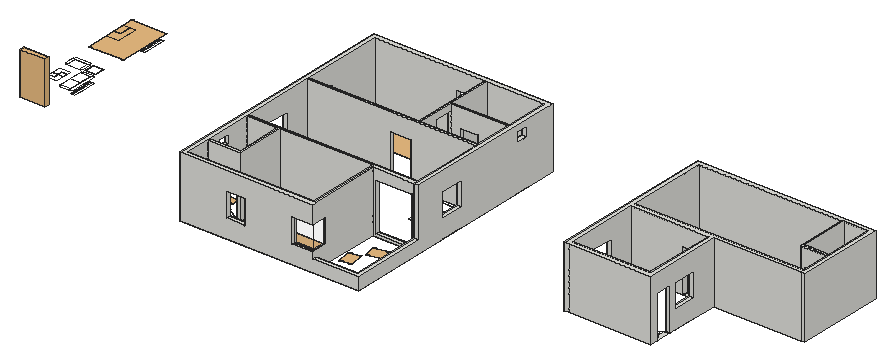
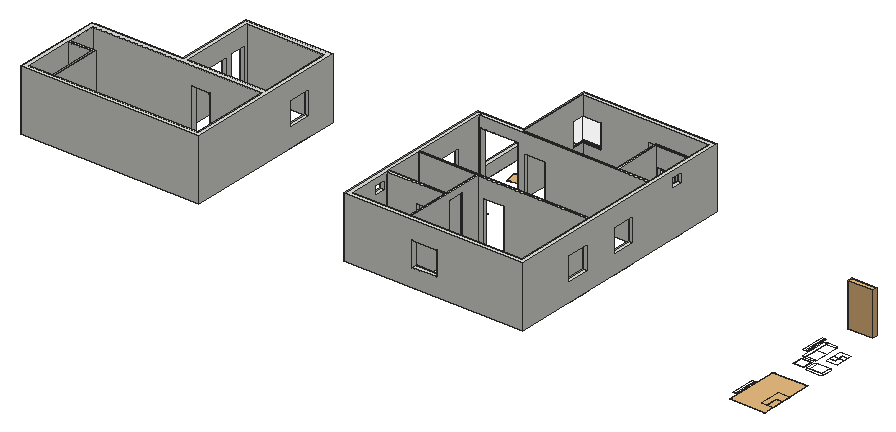
# SketchUp Ruby script. Lengths in inches.
U = 1.inch
M = Sketchup.active_model
def pt(a) = Geom::Point3d.new(a.map { |v| v * U })
def face(e, loops, mat)
  f = e.add_face(loops[0].map { |a| pt(a) })
  loops[1..].each { |l| e.add_face(l.map { |a| pt(a) }).erase! }
  f.material = f.back_material = mat if mat
  f
end
# faces: each face lists its corners as indices into pts; further lists are holes
def faces(e, pts, list, mat = nil) = list.each { |f| face(e, (f[0].is_a?(Array) ? f : [f]).map { |l| l.map { |i| pts[i] } }, mat) }
# xy, xz, yz: faces in a plane at the given z, y or x. An outline is a flat list of corners, or four numbers for a rectangle; further outlines are holes
def ring(l) = l.size == 4 ? [[l[0], l[1]], [l[2], l[1]], [l[2], l[3]], [l[0], l[3]]] : l.each_slice(2).to_a
def flat(e, list, mat, &to3) = list.each { |f| face(e, (f[0].is_a?(Array) ? f : [f]).map { |l| ring(l).map { |u, v| to3.(u, v) } }, mat) }
def xy(e, z, list, mat = nil) = flat(e, list, mat) { |x, y| [x, y, z] }
def xz(e, y, list, mat = nil) = flat(e, list, mat) { |x, z| [x, y, z] }
def yz(e, x, list, mat = nil) = flat(e, list, mat) { |y, z| [x, y, z] }
def lines(e, pts, list) = list.each { |a, b| e.add_line(pt(pts[a]), pt(pts[b])) }
# prism: a flat outline (further loops are holes) pulled along v
def prism(e, loops, v, mat = nil)
  f = face(e, loops, mat); d = Geom::Vector3d.new(v.map { |x| x * U })
  f.pushpull(f.normal.samedirection?(d) ? d.length : -d.length)
end
def box(e, o, s, mat = nil) = prism(e, [[o, [o[0] + s[0], o[1], o[2]], [o[0] + s[0], o[1] + s[1], o[2]], [o[0], o[1] + s[1], o[2]]]], [0, 0, s[2]], mat)
def at(x, y, z, deg = 0) = Geom::Transformation.translation(pt([x, y, z])) * Geom::Transformation.rotation(ORIGIN, Z_AXIS, deg.degrees)
def axes(o, x, y, z) = Geom::Transformation.new([*x, 0, *y, 0, *z, 0, *pt(o).to_a, 1])
def part(name) = M.definitions.add(name)
# library, detail: a bought-in or finely detailed component or shape, given as its bounding box
def library(name, o, s) = part(name).tap { |d| box(d.entities, o, s) }
def detail(e, o, s) = box(e.add_group.entities, o, s)
def put(e, d, t, mat = nil) = e.add_instance(d, t).tap { |i| i.material = mat if mat }
def group(e, t, mat = nil) = e.add_group.tap { |g| g.transformation = t; g.material = mat if mat }.entities
root = M.entities
M.materials.add("[Translucent Glass Gray]").color = [128, 128, 128]
M.materials["[Translucent Glass Gray]"].alpha = 0.1
c1 = part("TABLE 2")
p = [[18.6875,1.33,0],[-2.65,1.33,0],[-2.65,-10.67,0],[-18.65,-10.67,0],[-18.6875,10.67,0],[18.6875,10.67,0],
  [18.6875,0,0],[18.6875,-10.67,0],[-1.28,-10.67,0],[-1.28,0,0]]
lines(c1.entities,p,[[0,1],[1,2],[2,3],[3,4],[4,5],[5,0],[6,7],[7,8],[8,9],[9,6]])
c2 = part("A$C03AA15B9")
p = [[12,-9.82,0],[0,-9.82,0],[0,-0.97,0],[12,-0.97,0],[-1.19,-0.97,0],[-1.19,-10.64,0],
  [12,-10.64,0],[12,-19.5,0],[-12,-19.5,0],[-12,-0.97,0],[-12,9.45,0],[0,9.45,0],
  [0,0.22,0],[-12,0.22,0],[1.19,0.22,0],[1.19,10.64,0],[-12,10.64,0],[-12,19.5,0],
  [12,19.5,0],[12,0.22,0]]
lines(c2.entities,p,[[0,1],[1,2],[2,3],[3,0],[4,5],[5,6],[6,7],[7,8],[8,9],[9,4],[10,11],[11,12],
  [12,13],[13,10],[14,15],[15,16],[16,17],[17,18],[18,19],[19,14]])
c3 = part("A$C47E27A62")
p = [[17.04,-15,0],[-17.04,-15,0],[-17.04,-12,0],[17.04,8.51,0],[-17.04,8.51,0],[17.04,15,0],
  [-17.04,15,0],[13.4375,7.07,0],[-13.4375,7.07,0],[-17.04,9.96,0],[-19.5625,9.96,0],[-19.5625,-12,0],
  [-13.4375,-12,0],[-13.4375,8.51,0],[17.04,-12,0],[17.04,9.96,0],[19.5625,9.96,0],[19.5625,-12,0],
  [13.4375,-12,0],[13.4375,8.51,0]]
lines(c3.entities,p,[[0,1],[2,1],[3,4],[5,6],[7,8],[9,10],[6,4],[11,12],[8,12],[13,8],[10,11],[14,0],
  [15,16],[17,18],[19,18],[16,17],[5,3]])
c4 = library("A$Ccaaf8ce0",[-55.9,-35.68,0],[111.8,71.36,0.01])
c5 = library("Door 243 065",[-19.36,-2.49,0],[38.72,4.98,81.96])
c6 = part("A$C21FE29A1")
p = [[-10,-10,0],[10,-10,0],[10,10,0],[-10,10,0],[-11,-11,0],[11,-11,0],
  [11,11,0],[-11,11,0],[-12,-12,0],[12,-12,0],[12,12,0],[-12,12,0]]
lines(c6.entities,p,[[0,1],[1,2],[2,3],[3,0],[4,5],[5,6],[6,7],[7,4],[8,9],[9,10],[10,11],[11,8]])
c7 = part("A$C0E8E2537")
p = [[30.48,-15,0],[-30.48,-15,0],[-30.48,-12,0],[0,-15,0],[0,7.07,0],[30.48,8.51,0],
  [-30.48,8.51,0],[30.48,15,0],[-30.48,15,0],[26.875,7.07,0],[-26.875,7.07,0],[-30.48,9.96,0],
  [-33,9.96,0],[-33,-12,0],[-26.875,-12,0],[-26.875,8.51,0],[30.48,-12,0],[30.48,9.96,0],
  [33,9.96,0],[33,-12,0],[26.875,-12,0],[26.875,8.51,0]]
lines(c7.entities,p,[[0,1],[2,1],[3,4],[5,6],[7,8],[9,10],[11,12],[8,6],[13,14],[10,14],[15,10],[12,13],
  [16,0],[17,18],[19,20],[21,20],[18,19],[7,5]])
c8 = part("A$C63CB6BFC")
p = [[-24,-4.5,0],[24,-4.5,0],[24,0,0],[-24,0,0],[22.01,2.25,0],[1.02,2.25,0],
  [-0.96,2.25,0],[-22.01,2.25,0],[-0.96,4.5,0],[-0.96,0,0],[1.02,0,0],[1.02,4.5,0],
  [-22.01,0,0],[-22.01,4.5,0],[22.01,0,0],[24,4.5,0],[-24,4.5,0],[22.01,4.5,0]]
lines(c8.entities,p,[[0,1],[2,3],[4,5],[6,7],[8,9],[9,10],[10,11],[3,12],[12,13],[14,2],[15,16],[15,1],
  [16,0],[17,14]])
c9 = part("VEN")
p = [[-4.5,-11.98,0],[4.5,-11.98,0],[2.25,10,0],[2.25,-10,0],[0,-11.98,0],[0,11.98,0],
  [0,-10,0],[4.5,-10,0],[4.5,10,0],[0,10,0],[4.5,11.98,0],[-4.5,11.98,0]]
lines(c9.entities,p,[[0,1],[2,3],[4,5],[6,7],[8,9],[1,10],[0,11],[10,11]])
c10 = part("new bloSDFck")
p = [[-0.99,-2.25,0],[-22.01,-2.25,0],[-0.99,-4.5,0],[-0.99,0,0],[0.99,0,0],[0.99,-4.5,0],
  [-24,-4.5,0],[-24,0,0],[-22.01,0,0],[-22.01,-4.5,0],[22.01,-4.5,0],[22.01,0,0],
  [24,0,0],[24,-4.5,0],[24,4.5,0],[-24,4.5,0],[22.01,-2.25,0],[0.99,-2.25,0]]
lines(c10.entities,p,[[0,1],[2,3],[4,5],[6,7],[7,8],[8,9],[10,11],[11,12],[12,13],[13,6],[13,14],[6,15],
  [15,14],[12,7],[16,17]])
c11 = library("SH",[-3.77,-3.27,-0.25],[7.54,6.54,0.5])
c12 = library("A$C4D064DB7",[-6.63,-3.5625,0],[13.26,7.125,0.01])
c13 = library("A$C0124305E",[-7.81,-9.6,0],[15.62,19.2,0.01])
c14 = library("A$C7d9d00ca",[-6.89,-10.82,0],[13.78,21.65,0.01])
c15 = library("SOFA1",[-400.02,-350.02,0],[800.04,700.04,0.01])
c16 = library("HYUU",[-119.32,-134.74,0],[238.64,269.48,0.01])
c17 = library("CH",[-6.93,-9.5,0],[13.85,19,0.01])
c18 = part("FHHGGHHJ")
p = [[-7.07,-12.65,0],[-6.44,-13.01,0],[5.93,9.87,0],[5.46,10.12,0],[4.97,10.35,0],[4.49,10.58,0],
  [4,10.8,0],[3.5,11.01,0],[3,11.2,0],[2.5,11.39,0],[1.99,11.57,0],[1.48,11.74,0],
  [0.97,11.89,0],[0.45,12.04,0],[-0.07,12.18,0],[-0.59,12.3,0],[-1.11,12.42,0],[-1.64,12.52,0],
  [-2.17,12.62,0],[-2.7,12.7,0],[-3.23,12.78,0],[-3.76,12.84,0],[-4.3,12.89,0],[-4.83,12.93,0],
  [-5.37,12.96,0],[-5.91,12.98,0],[-6.44,12.99,0],[6.56,9.51,0],[8.43,8.43,0],[-6.43,-13,0],
  [-8.43,-13,0],[-8.43,-15,0],[-6.43,-15,0],[-6.43,15,0],[-8.43,15,0],[-8.43,13,0],
  [-6.43,13,0]]
lines(c18.entities,p,[[0,1],[2,3],[3,4],[4,5],[5,6],[6,7],[7,8],[8,9],[9,10],[10,11],[11,12],[12,13],
  [13,14],[14,15],[15,16],[16,17],[17,18],[18,19],[19,20],[20,21],[21,22],[22,23],[23,24],[24,25],
  [25,26],[27,28],[2,0],[27,2],[1,27],[29,30],[30,31],[31,32],[32,29],[33,34],[34,35],[35,36],
  [36,33]])
c19 = part("A$C231C625F")
p = [[-0.375,-18,0],[1.125,-18,0],[1.125,18,0],[-0.375,18,0],[-1.125,-27,0],[-0.375,-27,0],
  [-0.375,27,0],[-1.125,27,0]]
lines(c19.entities,p,[[0,1],[1,2],[2,3],[3,0],[4,5],[5,6],[6,7],[7,4]])
c20 = part("rjhj")
p = [[42.32,6,0],[42.32,-6,0],[-42.32,-6,0],[-42.32,6,0]]
lines(c20.entities,p,[[0,1],[1,2],[2,3],[3,0]])
put(c20.entities,c19,axes([-0.78,-4.875,0],[0,-1,0],[-1,0,0],[0,0,1]))
c21 = part("WINDOW W2")
p = [[18,-4.5,0],[-18,-4.5,0],[-18,0,0],[18,0,0],[-16.01,2.25,0],[-1.02,2.25,0],
  [0.96,2.25,0],[16.01,2.25,0],[0.96,4.5,0],[0.96,0,0],[-1.02,0,0],[-1.02,4.5,0],
  [18,4.5,0],[16.01,0,0],[16.01,4.5,0],[-16.01,4.5,0],[-16.01,0,0],[-18,4.5,0]]
lines(c21.entities,p,[[0,1],[2,3],[4,5],[6,7],[8,9],[9,10],[10,11],[12,3],[3,13],[13,14],[15,16],[16,2],
  [2,17],[17,12],[17,1],[12,0]])
c22 = library("C.BED",[-51.01,-44.97,0],[102.02,92.7,0.01])
c23 = library("A$C994c1a7f",[-51.01,-35.89,0],[102.02,71.78,0.01])
c24 = part("dd")
p = [[-6.52,11.67,0],[-5.95,12.01,0],[5.48,-9.11,0],[5.04,-9.34,0],[4.59,-9.56,0],[4.14,-9.77,0],
  [3.6875,-9.97,0],[3.23,-10.16,0],[2.77,-10.34,0],[2.31,-10.52,0],[1.84,-10.68,0],[1.37,-10.83,0],
  [0.89,-10.98,0],[0.42,-11.11,0],[-0.0625,-11.24,0],[-0.54,-11.36,0],[-1.03,-11.46,0],[-1.51,-11.5625,0],
  [-2,-11.65,0],[-2.49,-11.73,0],[-2.98,-11.79,0],[-3.47,-11.85,0],[-3.97,-11.9,0],[-4.46,-11.9375,0],
  [-4.96,-11.97,0],[-5.45,-11.98,0],[-5.95,-11.99,0],[6.05,-8.78,0],[7.79,-7.78,0],[-5.9375,12,0],
  [-7.79,12,0],[-7.79,13.85,0],[-5.9375,13.85,0],[-5.9375,-13.85,0],[-7.79,-13.85,0],[-7.79,-12,0],
  [-5.9375,-12,0]]
lines(c24.entities,p,[[0,1],[2,3],[3,4],[4,5],[5,6],[6,7],[7,8],[8,9],[9,10],[10,11],[11,12],[12,13],
  [13,14],[14,15],[15,16],[16,17],[17,18],[18,19],[19,20],[20,21],[21,22],[22,23],[23,24],[24,25],
  [25,26],[27,28],[2,0],[27,2],[1,27],[29,30],[30,31],[31,32],[32,29],[33,34],[34,35],[35,36],
  [36,33]])
c25 = library("A$Cc61c0c62",[-18,-10.05,0],[36,20.1,0.01])
c26 = library("Chair 1",[-14.77,-12,0],[29.54,23.99,0.01])
detail(root,[8921.35,957.82,16.75],[21.07,20.19,0.875])
put(root,c1,axes([8472.46,915.9,16.75],[0,1.125,0],[1.125,0,0],[0,0,1.125]))
put(root,c2,axes([8478.46,753.98,16.75],[-0.89319,0,0],[0,0.89319,0],[0,0,0.89319]))
put(root,c3,axes([8481.38,799.8,16.75],[0.89319,0,0],[0,0.89319,0],[0,0,0.89319]))
put(root,c4,axes([8495.4,904.52,16.75],[0,-0.95,0],[-0.95,0,0],[0,0,0.95]))
put(root,c5,axes([8501.91,666.64,16.68],[1.24138,0,0],[0,1.90527,0],[0,0,1.02567]))
put(root,c6,axes([8513.51,799.36,16.75],[0,-0.89319,0],[0.89319,0,0],[0,0,0.89319]))
put(root,c7,axes([8514.29,755.375,16.75],[0,0.89319,0],[0.89319,0,0],[0,0,0.89319]))
put(root,c8,axes([8534.94,913.98,16.75],[0,-1,0],[-1,0,0],[0,0,1]))
put(root,c8,axes([8534.94,742.9,16.75],[0,-1,0],[-1,0,0],[0,0,1]))
put(root,c9,axes([8915.06,610.95,16.75],[1,0,0],[0,-1,0],[0,0,1]))
put(root,c10,at(8915.06,742.9,16.75,90))
put(root,c8,at(8915.06,854.24,16.75,-90))
put(root,c11,axes([8922.84,647.89,17],[0,1.00172,0],[-1.00172,0,0],[0,0,1.00172]))
put(root,c12,at(8926.2,647.92,16.75,180))
put(root,c13,axes([8927.37,589,16.75],[-1,0,0],[0,1,0],[0,0,1]))
put(root,c14,axes([8930.39,612.4,16.75],[0,-1,0],[-1,0,0],[0,0,1]))
put(root,c15,axes([8931.3,894.34,16.75],[0,0.02981,0],[-0.02981,0,0],[0,0,0.02981]))
put(root,c15,axes([8931.57,938.85,16.75],[0,-0.02981,0],[-0.02981,0,0],[0,0,0.02981]))
put(root,c16,axes([8931.66,968.15,16.75],[0.08778,0,0],[0,0.08778,0],[0,0,0.08778]))
put(root,c17,axes([8942.875,542.65,16.75],[1.2,0,0],[0,1.2,0],[0,0,1.2]))
put(root,c18,axes([8958.56,581.18,16.75],[0,1.1,0],[-1.1,0,0],[0,0,1.1]))
put(root,c20,axes([9006.69,823.9,16.75],[-0.75,0,0],[0,0.75,0],[0,0,0.75]))
put(root,c21,at(9019.84,517.9,16.75))
put(root,c22,axes([9038.25,929.88,16.75],[-1,0,0],[0,1,0],[0,0,1]))
put(root,c23,at(9082.16,558.92,16.75))
g1 = group(root,at(8910.56,513.4,16.75))
xy(g1,0,[[[0,0,351,477],[9,9,342,468]],[256.5,9,256.5,153,252,153,252,157.5,342,157.5,342,148.5,261,148.5,261,9],[64.5,58.5,64.5,63,69,63,69,153,9,153,9,157.5,213,157.5,213,153,73.5,153,73.5,58.5],[9,58.5,31.5,63],[9,301.5,174,306],
  [213,301.5,213,306,225,306,225,342,229.5,342,229.5,306,342,306,342,301.5],[225,378,225,468,229.5,468,229.5,382.5,250.5,382.5,250.5,378],[283.5,378,342,382.5]])
xy(g1,4,[[265.5,148.5,337.5,157.5]])
xy(g1,23.5625,[[261,0,351,0,351,148.5,342,148.5,342,9,261,9]])
xy(g1,36,[[91.28,0,127.28,9],[220.5,0,261,0,261,33,258.75,33,258.75,4.5,220.5,4.5],[220.5,4.5,258.75,4.5,258.75,33,256.5,33,256.5,9,220.5,9],[0,205.5,9,253.5],[342,205.5,351,253.5],
  [0,316.84,9,364.84],[169.31,468,217.31,477]])
xy(g1,84,[[91.28,0,127.28,9],[220.5,0,220.5,4.5,258.75,4.5,258.75,33,261,33,261,0],[220.5,4.5,220.5,9,256.5,9,256.5,33,258.75,33,258.75,4.5],[31.5,58.5,64.5,63],[213,153,252,157.5],
  [0,205.5,9,253.5],[342,205.5,351,253.5],[174,301.5,213,306],[0,316.84,9,364.84],[250.5,378,283.5,382.5],
  [169.31,468,217.31,477]])
xy(g1,90,[[0,85.57,9,109.53],[342,389.07,351,413.03]])
xy(g1,100,[[265.5,148.5,337.5,157.5]])
xy(g1,108,[[0,85.57,9,109.53],[225,342,229.5,378],[342,389.07,351,413.03]])
xy(g1,120,[[0,0,261,0,261,148.5,342,148.5,342,157.5,9,157.5,9,153,69,153,69,63,9,63,9,58.5,73.5,58.5,73.5,153,256.5,153,256.5,9,9,9,9,468,342,468,342,148.5,351,148.5,351,477,0,477],[9,301.5,342,301.5,342,306,229.5,306,229.5,378,342,378,342,382.5,229.5,382.5,229.5,468,225,468,225,306,9,306]])
xz(g1,0,[[[0,0,351,0,351,23.5625,261,23.5625,261,36,220.5,36,220.5,84,261,84,261,120,0,120],[91.28,36,127.28,84]]])
xz(g1,4.5,[[220.5,36,258.75,84]],"[Translucent Glass Gray]")
xz(g1,9,[[[9,0,9,120,256.5,120,256.5,84,220.5,84,220.5,36,256.5,36,256.5,0],[91.28,36,127.28,84]],[261,0,342,23.5625]])
xz(g1,33,[[256.5,36,258.75,84],[258.75,36,261,84]])
xz(g1,58.5,[[9,0,31.5,0,31.5,84,64.5,84,64.5,0,73.5,0,73.5,120,9,120]])
xz(g1,63,[[9,0,9,120,69,120,69,0,64.5,0,64.5,84,31.5,84,31.5,0]])
xz(g1,85.57,[[0,90,9,108]])
xz(g1,109.53,[[0,90,9,108]])
xz(g1,148.5,[[[261,0,342,120],[265.5,4,337.5,100]],[342,23.5625,351,120]])
xz(g1,153,[[9,0,69,120],[73.5,0,213,0,213,84,252,84,252,0,256.5,0,256.5,120,73.5,120]])
xz(g1,157.5,[[[9,0,9,120,342,120,342,0,252,0,252,84,213,84,213,0],[265.5,4,337.5,100]]])
xz(g1,205.5,[[0,36,9,84],[342,36,351,84]])
xz(g1,253.5,[[0,36,9,84],[342,36,351,84]])
xz(g1,301.5,[[9,0,174,0,174,84,213,84,213,0,342,0,342,120,9,120]])
xz(g1,306,[[9,0,9,120,225,120,225,0,213,0,213,84,174,84,174,0],[229.5,0,342,120]])
xz(g1,316.84,[[0,36,9,84]])
xz(g1,342,[[225,0,229.5,108]])
xz(g1,364.84,[[0,36,9,84]])
xz(g1,378,[[225,0,229.5,108],[229.5,0,250.5,0,250.5,84,283.5,84,283.5,0,342,0,342,120,229.5,120]])
xz(g1,382.5,[[229.5,0,229.5,120,342,120,342,0,283.5,0,283.5,84,250.5,84,250.5,0]])
xz(g1,389.07,[[342,90,351,108]])
xz(g1,413.03,[[342,90,351,108]])
xz(g1,468,[[[9,0,225,120],[169.31,36,217.31,84]],[225,0,229.5,120],[229.5,0,342,120]])
xz(g1,477,[[[0,0,351,120],[169.31,36,217.31,84]]])
yz(g1,0,[[[0,0,477,120],[316.84,36,364.84,84],[205.5,36,253.5,84],[85.57,90,109.53,108]]])
yz(g1,9,[[9,0,58.5,120],[58.5,0,63,120],[[63,0,153,120],[85.57,90,109.53,108]],[153,0,157.5,120],[[157.5,0,301.5,120],[205.5,36,253.5,84]],
  [301.5,0,306,120],[[306,0,468,120],[316.84,36,364.84,84]]])
yz(g1,31.5,[[58.5,0,63,84]])
yz(g1,64.5,[[58.5,0,63,84]])
yz(g1,69,[[63,0,153,120]])
yz(g1,73.5,[[58.5,0,153,120]])
yz(g1,91.28,[[0,36,9,84]])
yz(g1,127.28,[[0,36,9,84]])
yz(g1,169.31,[[468,36,477,84]])
yz(g1,174,[[301.5,0,306,84]])
yz(g1,213,[[153,0,157.5,84],[301.5,0,306,84]])
yz(g1,217.31,[[468,36,477,84]])
yz(g1,220.5,[[0,36,4.5,84],[4.5,36,9,84]])
yz(g1,225,[[306,0,306,120,468,120,468,0,378,0,378,108,342,108,342,0]])
yz(g1,229.5,[[306,0,342,0,342,108,378,108,378,120,306,120],[382.5,0,468,120]])
yz(g1,250.5,[[378,0,382.5,84]])
yz(g1,252,[[153,0,157.5,84]])
yz(g1,256.5,[[9,0,9,36,33,36,33,84,9,84,9,120,153,120,153,0]])
yz(g1,258.75,[[4.5,36,33,84]],"[Translucent Glass Gray]")
yz(g1,261,[[9,0,148.13,0,148.13,120,0,120,0,84,33,84,33,36,0,36,0,23.5625,9,23.5625],[148.13,0,148.5,120]])
yz(g1,265.5,[[148.5,4,157.5,100]])
yz(g1,283.5,[[378,0,382.5,84]])
yz(g1,337.5,[[148.5,4,157.5,100]])
yz(g1,342,[[9,0,148.5,23.5625],[148.5,0,157.5,120],[[157.5,0,301.5,120],[205.5,36,253.5,84]],[301.5,0,306,120],[306,0,378,120],
  [378,0,382.5,120],[[382.5,0,468,120],[389.07,90,413.03,108]]])
yz(g1,351,[[[0,0,477,0,477,120,148.5,120,148.5,23.5625,0,23.5625],[205.5,36,253.5,84],[389.07,90,413.03,108]]])
put(root,c8,axes([9103.87,985.9,16.75],[1,0,0],[0,-1,0],[0,0,1]))
put(root,c24,axes([9104.06,825.87,16.75],[0,1.40833,0],[1.40833,0,0],[0,0,1.40833]))
put(root,c24,axes([9143.06,659.94,16.75],[0,-1.40833,0],[1.40833,0,0],[0,0,1.40833]))
put(root,c25,at(9172.01,971.35,16.75,180))
put(root,c18,axes([9177.56,900.68,16.75],[0,1.1,0],[1.1,0,0],[0,0,1.1]))
put(root,c26,at(9188.93,583.87,16.75,100.137))
put(root,c2,axes([9191.87,753.32,16.75],[0.89319,0,0],[0,0.89319,0],[0,0,0.89319]))
put(root,c7,axes([9191.89,801.51,16.75],[0.89319,0,0],[0,0.89319,0],[0,0,0.89319]))
put(root,c26,axes([9213.37,622.3125,16.75],[-0.97777,-0.2097,0],[-0.2097,0.97777,0],[0,0,1]))
put(root,c17,axes([9229.25,867.54,16.75],[-1.2,0,0],[0,-1.2,0],[0,0,1.2]))
put(root,c6,axes([9236.81,801.87,16.75],[-0.89319,0,0],[0,0.89319,0],[0,0,0.89319]))
put(root,c3,axes([9237.61,733.98,16.75],[0,0.89319,0],[0.89319,0,0],[0,0,0.89319]))
put(root,c3,axes([9237.61,768.93,16.75],[0,0.89319,0],[0.89319,0,0],[0,0,0.89319]))
put(root,c14,axes([9241.73,915.83,16.75],[0,1,0],[1,0,0],[0,0,1]))
put(root,c12,at(9245.93,960.94,16.75))
put(root,c11,axes([9249.28,960.97,17],[0,-1.00172,0],[1.00172,0,0],[0,0,1.00172]))
put(root,c8,axes([9257.06,742.9,16.75],[0,-1,0],[-1,0,0],[0,0,1]))
put(root,c9,at(9257.06,914.45,16.75,180))
put(root,c10,at(9552,742.9,16.75,90))
put(root,c20,axes([9561,903,16.75],[0,0.75,0],[0.75,0,0],[0,0,0.75]))
put(root,c18,axes([9676.34,825.03,16.75],[0,1.2,0],[-1.2,0,0],[0,0,1.2]))
put(root,c24,axes([9709.23,691.9,16.75],[-1.19167,0,0],[0,-1.19167,0],[0,0,1.19167]))
put(root,c8,axes([9714,742.9,16.75],[0,-1,0],[-1,0,0],[0,0,1]))
g2 = group(root,at(9547.5,513.4,16.75))
xy(g2,0,[[162,162,171,195],[110.84,301.5,146.84,310.5],[298.5,367.5,331.5,372]])
xy(g2,36,[[0,205.5,9,253.5],[162,205.5,171,253.5]])
xy(g2,84,[[162,162,171,195],[0,205.5,9,253.5],[162,205.5,171,253.5],[110.84,301.5,146.84,310.5],[298.5,367.5,331.5,372]])
xy(g2,120,[[[0,148.5,171,148.5,171,301.5,351,301.5,351,477,0,477],[9,310.5,9,468,342,468,342,372,294,372,294,468,289.5,468,289.5,367.5,342,367.5,342,310.5],[9,157.5,162,301.5]]])
xz(g2,148.5,[[0,0,9,120],[9,0,171,120]])
xz(g2,157.5,[[9,0,162,120]])
xz(g2,162,[[162,0,171,84]])
xz(g2,195,[[162,0,171,84]])
xz(g2,205.5,[[0,36,9,84],[162,36,171,84]])
xz(g2,253.5,[[0,36,9,84],[162,36,171,84]])
xz(g2,301.5,[[9,0,110.84,0,110.84,84,146.84,84,146.84,0,162,0,162,120,9,120],[171,0,342,120],[342,0,351,120]])
xz(g2,310.5,[[9,0,9,120,342,120,342,0,146.84,0,146.84,84,110.84,84,110.84,0]])
xz(g2,367.5,[[289.5,0,298.5,0,298.5,84,331.5,84,331.5,0,342,0,342,120,289.5,120]])
xz(g2,372,[[294,0,294,120,342,120,342,0,331.5,0,331.5,84,298.5,84,298.5,0]])
xz(g2,468,[[9,0,289.5,120],[289.5,0,294,120],[294,0,342,120]])
xz(g2,477,[[0,0,351,120]])
yz(g2,0,[[[148.5,0,477,120],[205.5,36,253.5,84]]])
yz(g2,9,[[[157.5,0,301.5,120],[205.5,36,253.5,84]],[310.5,0,468,120]])
yz(g2,110.84,[[301.5,0,310.5,84]])
yz(g2,146.84,[[301.5,0,310.5,84]])
yz(g2,162,[[[157.5,0,157.5,120,301.5,120,301.5,0,195,0,195,84,162,84,162,0],[205.5,36,253.5,84]]])
yz(g2,171,[[[148.5,0,162,0,162,84,195,84,195,0,301.5,0,301.5,120,148.5,120],[205.5,36,253.5,84]]])
yz(g2,289.5,[[367.5,0,468,120]])
yz(g2,294,[[372,0,468,120]])
yz(g2,298.5,[[367.5,0,372,84]])
yz(g2,331.5,[[367.5,0,372,84]])
yz(g2,342,[[310.5,0,367.5,120],[372,0,468,120]])
yz(g2,351,[[301.5,0,477,120]])
# 6 loose lines left out
put(root,c18,axes([9862.5,890.18,16.75],[0,1.1,0],[1.1,0,0],[0,0,1.1]))
